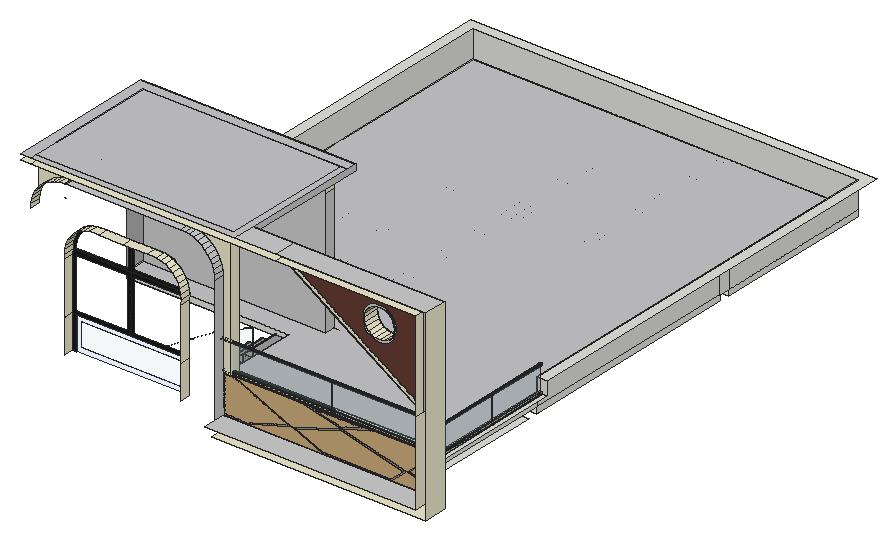
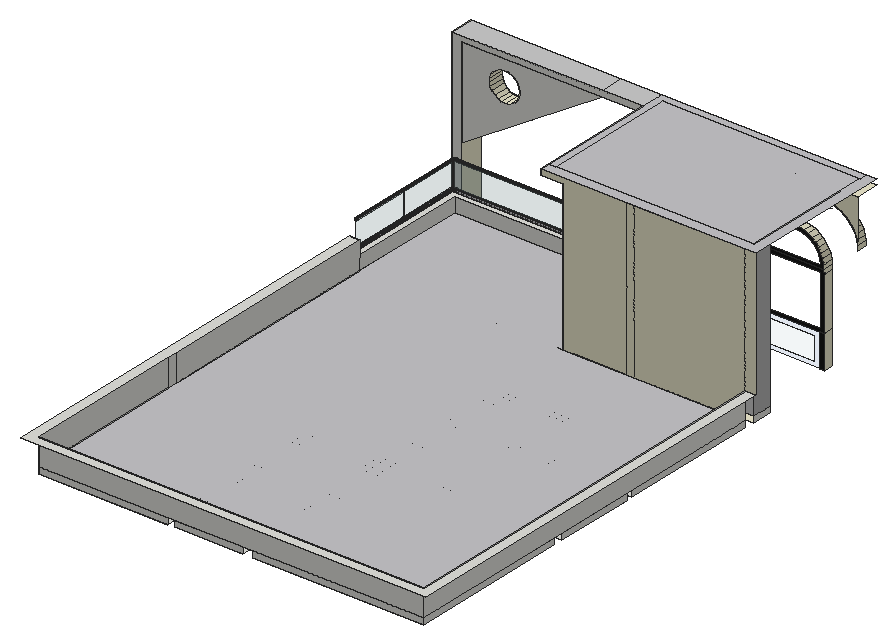
# SketchUp Ruby script. Lengths in inches.
U = 1.inch
M = Sketchup.active_model
def pt(a) = Geom::Point3d.new(a.map { |v| v * U })
def face(e, loops, mat)
  f = e.add_face(loops[0].map { |a| pt(a) })
  loops[1..].each { |l| e.add_face(l.map { |a| pt(a) }).erase! }
  f.material = f.back_material = mat if mat
  f
end
# faces: each face lists its corners as indices into pts; further lists are holes
def faces(e, pts, list, mat = nil) = list.each { |f| face(e, (f[0].is_a?(Array) ? f : [f]).map { |l| l.map { |i| pts[i] } }, mat) }
# xy, xz, yz: faces in a plane at the given z, y or x. An outline is a flat list of corners, or four numbers for a rectangle; further outlines are holes
def ring(l) = l.size == 4 ? [[l[0], l[1]], [l[2], l[1]], [l[2], l[3]], [l[0], l[3]]] : l.each_slice(2).to_a
def flat(e, list, mat, &to3) = list.each { |f| face(e, (f[0].is_a?(Array) ? f : [f]).map { |l| ring(l).map { |u, v| to3.(u, v) } }, mat) }
def xy(e, z, list, mat = nil) = flat(e, list, mat) { |x, y| [x, y, z] }
def xz(e, y, list, mat = nil) = flat(e, list, mat) { |x, z| [x, y, z] }
def yz(e, x, list, mat = nil) = flat(e, list, mat) { |y, z| [x, y, z] }
def lines(e, pts, list) = list.each { |a, b| e.add_line(pt(pts[a]), pt(pts[b])) }
# prism: a flat outline (further loops are holes) pulled along v
def prism(e, loops, v, mat = nil)
  f = face(e, loops, mat); d = Geom::Vector3d.new(v.map { |x| x * U })
  f.pushpull(f.normal.samedirection?(d) ? d.length : -d.length)
end
def box(e, o, s, mat = nil) = prism(e, [[o, [o[0] + s[0], o[1], o[2]], [o[0] + s[0], o[1] + s[1], o[2]], [o[0], o[1] + s[1], o[2]]]], [0, 0, s[2]], mat)
def at(x, y, z, deg = 0) = Geom::Transformation.translation(pt([x, y, z])) * Geom::Transformation.rotation(ORIGIN, Z_AXIS, deg.degrees)
def axes(o, x, y, z) = Geom::Transformation.new([*x, 0, *y, 0, *z, 0, *pt(o).to_a, 1])
def part(name) = M.definitions.add(name)
# library, detail: a bought-in or finely detailed component or shape, given as its bounding box
def library(name, o, s) = part(name).tap { |d| box(d.entities, o, s) }
def detail(e, o, s) = box(e.add_group.entities, o, s)
def put(e, d, t, mat = nil) = e.add_instance(d, t).tap { |i| i.material = mat if mat }
def group(e, t, mat = nil) = e.add_group.tap { |g| g.transformation = t; g.material = mat if mat }.entities
root = M.entities
M.materials.add("Copper (DK9VGZ)").color = [173, 110, 84]
M.materials.add("Distressed Leather (CCZUWY)").color = [102, 60, 53]
M.materials.add("Drag Textured Plaster None 1500 x 1662 mm (I93S2X)").color = [206, 173, 125]
M.materials.add("Drag Textured Plaster None 1500 x 1662 mm (TE616Y)").color = [206, 173, 125]
M.materials.add("Grey4").color = [61, 61, 61]
M.materials.add("Lily_Blonde").color = [237, 233, 206]
M.materials.add("Rosso Verona Marble Herringbone 1146 x 891 mm (N04GW4)").color = [204, 94, 55]
M.materials.add("Rust-Stain-Remover").color = [206, 203, 196]
M.materials["Rust-Stain-Remover"].alpha = 0.13
M.materials.add("Textured Stucco (8DUEUS)").color = [204, 204, 204]
M.materials.add("Wood Wool (CH8A6D)").color = [158, 148, 138]
M.materials.add("[0136_Charcoal]").color = [25, 25, 25]
M.materials.add("[Aluminum]").color = [178, 178, 178]
M.materials.add("[Metal Silver]").color = [198, 197, 201]
M.materials.add("[Metal Silver]1").color = [234, 233, 238]
M.materials.add("[Translucent Glass Blue]1").color = [97, 145, 232]
M.materials["[Translucent Glass Blue]1"].alpha = 0.15
M.materials.add("[Translucent Glass Gray]").color = [73, 161, 170]
M.materials["[Translucent Glass Gray]"].alpha = 0.06
M.materials.add("crushed-stone-asphalt-staggered-isosceles-2423-mm-architextu").color = [158, 158, 157]
c1 = part("Stair tread")
xy(c1.entities,0,[[0,0,11.5,36]])
xy(c1.entities,7,[[0,0,11.5,36]])
xz(c1.entities,0,[[0,0,11.5,7],[11.5,6,11.63,6.02,11.75,6.07,11.85,6.15,11.93,6.25,11.98,6.37,12,6.5,11.98,6.63,11.93,6.75,11.85,6.85,11.75,6.93,11.63,6.98,11.5,7]])
xz(c1.entities,36,[[0,0,11.5,7],[11.5,6,11.5,7,11.63,6.98,11.75,6.93,11.85,6.85,11.93,6.75,11.98,6.63,12,6.5,11.98,6.37,11.93,6.25,11.85,6.15,11.75,6.07,11.63,6.02]])
yz(c1.entities,0,[[0,0,36,7]])
yz(c1.entities,11.5,[[0,0,36,6],[0,6,10.3125,7],[10.3125,6,36,7]])
p = [[11.5,36,6],[11.63,36,6.02],[11.63,0,6.02],[11.5,0,6],[11.5,10.3125,6],[11.75,36,6.07],
  [11.75,0,6.07],[11.85,36,6.15],[11.85,0,6.15],[11.93,36,6.25],[11.93,0,6.25],[11.98,36,6.37],
  [11.98,0,6.37],[12,36,6.5],[12,0,6.5],[11.98,36,6.63],[11.98,0,6.63],[11.93,36,6.75],
  [11.93,0,6.75],[11.85,36,6.85],[11.85,0,6.85],[11.75,36,6.93],[11.63,36,6.98],[11.63,0,6.98],
  [11.75,0,6.93],[11.5,36,7],[11.5,10.3125,7],[11.5,0,7]]
faces(c1.entities,p,[[0,1,2,3,4],[1,5,6,2],[5,7,8,6],[7,9,10,8],[9,11,12,10],[11,13,14,12],[13,15,16,14],[15,17,18,16],
  [17,19,20,18],[21,22,23,24],[19,21,24,20],[25,26,27,23,22]])
c2 = part("Группа\#2")
box(c2.entities,[0,0,0],[41.85,0.39,23.61])
c3 = part("Группа\#3")
prism(c3.entities,[[[0,1.0625,0],[0,0.09,0],[0,0,0.09],[0,0,0.56],[0,0.2,0.66],[0,0.06,0.66],[0,0,0.72],[0,0,2.28],[0,0.4,2.69],[0,0.74,2.69],[0,0.74,1.08],[0,1.0625,1.08],[0,1.39,1.08],[0,1.39,2.69],[0,1.6875,2.69],[0,1.85,2.48],[0,1.85,0.09],[0,1.76,0]]],[41.85,0,0])
c4 = part("Группа\#4")
xy(c4.entities,0,[[0,0.06,41.85,0.58]],"[0136_Charcoal]")
xy(c4.entities,0.12,[[0,0.11,41.85,0.54]],"[Metal Silver]1")
xz(c4.entities,0,[[0,0.06,41.85,1.61]],"[0136_Charcoal]")
xz(c4.entities,0.11,[[0,0.12,41.85,1.67]],"[0136_Charcoal]")
xz(c4.entities,0.54,[[0,0.12,41.85,1.67]],"[0136_Charcoal]")
xz(c4.entities,0.65,[[0,0.07,41.85,1.61]],"[0136_Charcoal]")
yz(c4.entities,0,[[0.06,0,0,0.06,0,1.61,0.11,1.67,0.11,0.12,0.54,0.12,0.54,1.67,0.65,1.61,0.65,0.07,0.58,0]],"[0136_Charcoal]")
yz(c4.entities,41.85,[[0.06,0,0.58,0,0.65,0.07,0.65,1.61,0.54,1.67,0.54,0.12,0.11,0.12,0.11,1.67,0,1.61,0,0.06]],"[0136_Charcoal]")
p = [[41.85,0.06,0],[41.85,0,0.06],[0,0,0.06],[0,0.06,0],[41.85,0.65,0.07],[41.85,0.58,0],
  [0,0.58,0],[0,0.65,0.07],[41.85,0,1.61],[41.85,0.11,1.67],[0,0.11,1.67],[0,0,1.61],
  [41.85,0.54,1.67],[41.85,0.65,1.61],[0,0.65,1.61],[0,0.54,1.67]]
faces(c4.entities,p,[[0,1,2,3],[4,5,6,7],[8,9,10,11],[12,13,14,15]],"[0136_Charcoal]")
c5 = part("Группа\#5")
prism(c5.entities,[[[0,0.73,0],[0,0.49,0.1],[0,0.29,0.25],[0,0.13,0.46],[0,0.03,0.7],[0,0,0.95],[0,0.03,1.21],[0,0.13,1.44],[0,0.29,1.65],[0,0.49,1.8],[0,0.73,1.9],[0,0.98,1.93],[0,1.24,1.9],[0,1.48,1.8],[0,1.68,1.65],[0,1.84,1.44],[0,1.93,1.21],[0,1.97,0.95],[0,1.93,0.7],[0,1.84,0.46],[0,1.68,0.25],[0,1.48,0.1],[0,1.24,0],[0,1.24,0.55],[0,0.73,0.55]]],[83.93,0,0])
c6 = part("Группа\#1")
xz(c6.entities,0,[[0,0,41.85,23.61]],"Rust-Stain-Remover")
c7 = part("Группа\#6")
xz(c7.entities,0,[[0,0,41.85,23.61]],"Rust-Stain-Remover")
c8 = part("Перила_14")
put(c8.entities,c2,at(0,-0.2,1.22),"[Translucent Glass Gray]")
put(c8.entities,c3,at(0,-1.0625,0),"[Metal Silver]")
put(c8.entities,c4,at(0,-0.32,1.08))
put(c8.entities,c5,at(0,-0.98,24.31),"[Metal Silver]1")
put(c8.entities,c6,at(0,0,1.22))
put(c8.entities,c4,at(42.09,-0.32,1.08))
put(c8.entities,c2,at(42.09,-0.2,1.22),"[Translucent Glass Gray]")
put(c8.entities,c3,at(42.09,-1.0625,0),"[Metal Silver]")
put(c8.entities,c7,at(42.09,0,1.22))
xy(root,132.6875,[[163.71,20.75,281.1875,29.1875]])
xy(root,132.8125,[[169.71,0,360,20.75]],"Lily_Blonde")
xy(root,138.8125,[[163.71,0,351.58,20.75]],"Textured Stucco (8DUEUS)")
xy(root,156,[[163.71,29.1875,163.71,29.25,152.42,29.25,152.42,125.1875,351,125.1875,351,29.1875],[9,134.1875,9,260.1875,78,260.1875,78,266.1875,9,266.1875,9,338.1875,108,338.1875,108,260.1875,170,260.1875,170,302.1875,161,302.1875,161,266.1875,114,266.1875,114,338.1875,161,338.1875,161,332.1875,170,332.1875,170,338.1875,176,338.1875,176,347.1875,170,347.1875,170,353.1875,161,353.1875,161,347.1875,9,347.1875,9,491.1875,161,491.1875,161,395.1875,170,395.1875,170,416.1875,230,416.1875,230,395.1875,236,395.1875,236,455.1875,230,455.1875,230,422.1875,170,422.1875,170,491.1875,230,491.1875,230,485.1875,236,485.1875,236,491.1875,351,491.1875,351,347.1875,236,347.1875,236,353.1875,230,353.1875,230,338.1875,351,338.1875,351,134.1875,170,134.1875,170,224.1875,161,224.1875,161,213.1875,155,213.1875,155,207.1875,161,207.1875,161,134.1875,114,134.1875,114,207.1875,120,207.1875,120,213.1875,108,213.1875,108,134.1875]])
xy(root,156,[[9,107.1875,152.42,125.1875]],"Lily_Blonde")
xy(root,157.02,[[140.92,70.6875,149.67,71.1875]])
xy(root,161,[[163.71,29.1875,351,29.1875,351,491.1875,9,491.1875,9,134.1875,170.71,134.1875,170.71,125.1875,9,125.1875,9,107.1875,152.42,107.1875,152.42,29.25,163.71,29.25]],"[Metal Silver]")
xy(root,173,[[163.71,20.75,170.71,29.1875],[170.71,20.75,360,20.75,360,134.1875,351,134.1875,351,29.1875,170.71,29.1875]])
xy(root,173,[[163.71,20.1875,170.71,20.75]],"Grey4")
xy(root,185,[[0,134.1875,9,134.1875,9,491.1875,351,491.1875,351,134.1875,360,134.1875,360,500.1875,0,500.1875]])
xy(root,250,[[52.44,11.4375,60.625,20.1875],[60.625,11.4375,82.18,20.1875],[82.18,11.4375,103.73,20.1875],[103.73,11.4375,111.91,20.1875]],"Lily_Blonde")
xy(root,279.9375,[[154.71,29.1875,152,125.1875,170.71,125.1875,170.71,29.1875]])
xy(root,280,[[30,11.4375,30.32,20.1875],[30.32,11.4375,31.32,20.1875]],"Copper (DK9VGZ)")
xy(root,280,[[31.32,11.4375,133.71,20.1875]],"Textured Stucco (8DUEUS)")
xy(root,293,[[9,29.1875,9,125.1875,152,125.1875,154.71,29.1875]])
xy(root,293,[[0,0,9,20.1875],[9,0,226.71,20.1875],[226.71,0,351.58,6.9375],[170.71,20.1875,170.71,134.1875,190.71,134.1875,190.71,20.75,226.71,20.75,226.71,20.1875]],"Lily_Blonde")
xy(root,293,[[226.71,6.9375,351.58,20.75]],"Textured Stucco (8DUEUS)")
xy(root,298,[[190.71,0,226.71,20.75],[226.71,0,360,20.75]],"Textured Stucco (8DUEUS)")
xy(root,298,[[0,0,9,0,9,125.1875,190.71,125.1875,190.71,134.1875,0,134.1875],[9,0,190.71,0,190.71,125.1875,184.71,125.1875,184.71,6,9,6],[9,6,184.71,125.1875]],"[Metal Silver]")
xz(root,6.9375,[[[348.16,218.71,348.16,289.58,238.32,289.58],[312.95,255,309.01,255.67,305.37,257.33,302.29,259.88,299.98,263.14,298.59,266.89,298.22,270.87,298.89,274.8125,300.56,278.45,303.11,281.52,306.37,283.84,310.11,285.23,314.09,285.6,318.03,284.93,321.67,283.26,324.75,280.71,327.06,277.45,328.45,273.7,328.82,269.72,328.15,265.78,326.49,262.15,323.93,259.07,320.67,256.76,316.93,255.37]]],"Distressed Leather (CCZUWY)")
xz(root,6.9375,[[[351.58,212.4375,351.58,293,226.71,293,289.14,252.72],[348.16,218.71,238.32,289.58,348.16,289.58]]],"Lily_Blonde")
xz(root,6.9375,[[[312.95,255,316.93,255.37,320.67,256.76,323.93,259.07,326.49,262.15,328.15,265.78,328.82,269.72,328.45,273.7,327.06,277.45,324.75,280.71,321.67,283.26,318.03,284.93,314.09,285.6,310.11,285.23,306.37,283.84,303.11,281.52,300.56,278.45,298.89,274.8125,298.22,270.87,298.59,266.89,299.98,263.14,302.29,259.88,305.37,257.33,309.01,255.67],[313.02,256.93,309.58,257.51,306.4,258.97,303.71,261.2,301.69,264.05,300.48,267.32,300.15,270.8,300.74,274.24,302.19,277.42,304.42,280.11,307.27,282.13,310.54,283.34,314.02,283.67,317.46,283.08,320.64,281.625,323.33,279.4,325.35,276.55,326.5625,273.27,326.89,269.8,326.31,266.35,324.85,263.18,322.62,260.49,319.77,258.47,316.5,257.25]]],"Textured Stucco (8DUEUS)")
xz(root,20.1875,[[163.71,173,170.71,173,170.71,293,0,293,0,250,0.26,253.92,1.02,257.76,2.28,261.48,4.02,265,6.2,268.26,8.79,271.21,11.74,273.8,15,275.98,18.52,277.72,22.24,278.98,26.08,279.74,30,280,133.71,280,137.625,279.74,141.47,278.98,145.1875,277.72,148.71,275.98,151.97,273.8,154.92,271.21,157.51,268.26,159.6875,265,161.42,261.48,162.69,257.76,163.45,253.92,163.71,250]],"Lily_Blonde")
xz(root,20.1875,[[30,144,33.9,173],[130.23,144,133.71,173],[[30,173,82.18,173,82.18,224.1,30.32,224.1,30,220],[33.15,176.15,33.15,219.875,33.24,220.95,79.02,220.95,79.02,176.15]],[[82.18,173,133.71,173,133.71,220,134.03,224.1,82.18,224.1],[85.05,175.87,85.05,221.23,130.92,221.23,130.84,220.11,130.84,175.87]],[[30.32,224.1,82.18,224.1,82.18,250,52.44,250,48.44,249.04,44.64,247.47,41.13,245.32,38,242.65,35.33,239.52,33.18,236.01,31.61,232.21,30.65,228.2],[32.64,226.25,32.77,227.87,33.65,231.54,35.1,235.03,37.07,238.25,39.52,241.125,42.4,243.58,45.62,245.55,49.11,247,52.7,247.86,80.03,247.86,80.03,226.25]],
  [[82.18,224.1,134.03,224.1,133.71,228.2,132.75,232.21,131.18,236.01,129.03,239.52,126.35,242.65,123.22,245.32,119.72,247.47,115.91,249.04,111.91,250,82.18,250],[84.45,226.375,84.45,247.73,111.64,247.73,115.21,246.875,118.68,245.4375,121.88,243.47,124.74,241.03,127.18,238.18,129.14,234.97,130.58,231.5,131.46,227.85,131.57,226.375]]],"[0136_Charcoal]")
xz(root,20.1875,[[[33.9,144,130.23,173],[38.1875,148.28,125.95,168.72]]],"[Translucent Glass Blue]1")
xz(root,20.1875,[[38.1875,148.28,125.95,168.72]],"[Translucent Glass Gray]")
xz(root,20.75,[[351.58,173,351.58,293,190.71,293,190.71,298,360,298,360,173],[[351.58,212.4375,289.14,252.72,226.71,293,351.58,293],[313.02,256.93,316.5,257.25,319.77,258.47,322.62,260.49,324.85,263.18,326.31,266.35,326.89,269.8,326.5625,273.27,325.35,276.55,323.33,279.4,320.64,281.625,317.46,283.08,314.02,283.67,310.54,283.34,307.27,282.13,304.42,280.11,302.19,277.42,300.74,274.24,300.15,270.8,300.48,267.32,301.69,264.05,303.71,261.2,306.4,258.97,309.58,257.51]]])
xz(root,20.75,[[184.63,138.8125,251.86,138.8125,224.17,150.92],[313.3,138.8125,351.58,138.8125,351.58,144.47,326.39,150.51],[164.7,139.81,184.48,139.81,221.3,151.09,173.46,172,164.7,172],[252.17,140.28,312.74,140.28,323.33,149.74,268.34,162.92,228.38,150.68],[350.65,145.65,350.65,170.93,328.33,151],
  [326.39,150.51,351.58,173,296.25,173,268.29,164.4375],[224.17,150.92,268.29,164.4375,232.57,173,173.67,173],[268.25,165.77,287.63,171.71,243.49,171.71]],"Drag Textured Plaster None 1500 x 1662 mm (I93S2X)")
xz(root,20.75,[[163.71,132.6875,169.71,132.6875,169.71,132.8125,360,132.8125,360,173,351.58,173,351.58,138.8125,163.71,138.8125]],"Drag Textured Plaster None 1500 x 1662 mm (TE616Y)")
xz(root,20.75,[[[163.71,138.8125,184.63,138.8125,224.17,150.92,173.67,173,163.71,173],[164.7,139.81,164.7,172,173.46,172,221.3,151.09,184.48,139.81]],[[251.86,138.8125,313.3,138.8125,326.39,150.51,268.29,164.4375,224.17,150.92],[252.17,140.28,228.38,150.68,268.34,162.92,323.33,149.74,312.74,140.28]],[[351.58,144.47,351.58,173,326.39,150.51],[350.65,145.65,328.33,151,350.65,170.93]],[[268.29,164.4375,296.25,173,232.57,173],[268.25,165.77,243.49,171.71,287.63,171.71]]],"Wood Wool (CH8A6D)")
xz(root,29.1875,[[163.71,132.6875,351,156],[163.71,161,351,173]])
xz(root,29.1875,[[163.71,173,170.71,279.9375]],"Grey4")
xz(root,29.25,[[152.42,156,163.71,161]])
xz(root,70.6875,[[117.92,143.04,140.92,157.02,149.67,157.02,149.67,181.02,117.92,167.02]],"[Translucent Glass Gray]")
xz(root,107.1875,[[9,156,152.42,161]])
xz(root,125.1875,[[9,161,170.71,161,170.71,279.9375,152,279.9375,152,293,9,293]],"Textured Stucco (8DUEUS)")
xz(root,134.1875,[[9,156,108,161],[114,156,161,161],[351,173,360,185]])
xz(root,134.1875,[[9,161,108,298],[108,161,114,298],[114,161,114,298,190.71,298,190.71,293,170.71,293,170.71,161],[0,185,9,298]],"Lily_Blonde")
xz(root,491.1875,[[9,156,161,161],[170,156,230,161],[236,156,351,161],[9,161,351,185]])
yz(root,9,[[107.1875,156,125.1875,161],[134.1875,156,260.1875,161],[266.1875,156,338.1875,161],[347.1875,156,491.1875,161],[134.1875,161,491.1875,185],
  [29.1875,293,107.1875,298],[107.1875,293,125.1875,298]])
yz(root,9,[[107.1875,161,125.1875,293]],"[Aluminum]")
yz(root,30,[[11.4375,144,20.1875,173],[11.4375,173,20.1875,220]],"Lily_Blonde")
yz(root,133.71,[[11.4375,144,20.1875,173],[11.4375,173,20.1875,220]],"Lily_Blonde")
yz(root,149.67,[[70.6875,157.02,71.1875,181.02]])
yz(root,152.42,[[29.25,156,107.1875,157.02],[29.25,157.02,107.1875,161]])
yz(root,163.71,[[20.75,144.15,29.1875,173],[29.1875,156,29.25,161]])
yz(root,163.71,[[20.75,132.6875,29.1875,144.15]],"Rosso Verona Marble Herringbone 1146 x 891 mm (N04GW4)")
yz(root,163.71,[[11.4375,138.8125,20.75,138.8125,20.75,173,20.1875,173,20.1875,250,11.4375,250]],"Textured Stucco (8DUEUS)")
yz(root,170.71,[[20.1875,173,29.1875,173,29.1875,279.9375,125.1875,279.9375,125.1875,271.4375,134.1875,271.4375,134.1875,293,20.1875,293]],"Lily_Blonde")
yz(root,170.71,[[125.1875,161,134.1875,271.4375]],"Textured Stucco (8DUEUS)")
yz(root,190.71,[[20.75,293,134.1875,298]],"Textured Stucco (8DUEUS)")
yz(root,351,[[134.1875,156,338.1875,161],[347.1875,156,491.1875,161],[29.1875,161,134.1875,173],[134.1875,161,338.1875,185],[338.1875,161,347.1875,185],
  [347.1875,161,491.1875,185]])
yz(root,351.58,[[0,138.8125,20.75,212.4375],[0,212.4375,6.9375,293]],"Lily_Blonde")
yz(root,351.58,[[6.9375,212.4375,20.75,293]],"Textured Stucco (8DUEUS)")
yz(root,360,[[0,132.8125,20.75,298]],"Lily_Blonde")
p = [[94.82,71.1875,153],[71.92,71.1875,139.02],[71.92,70.6875,139.02],[94.82,70.6875,153],[117.92,71.1875,143.04],[140.92,71.1875,157.02],
  [140.92,70.6875,157.02],[117.92,70.6875,143.04],[117.92,71.1875,167.02],[117.92,70.6875,167.02],[149.67,71.1875,181.02],[149.67,70.6875,181.02],
  [351.58,6.9375,212.4375],[289.14,6.9375,252.72],[289.14,20.75,252.72],[351.58,20.75,212.4375],[30,20.1875,220],[30.32,20.1875,224.1],
  [30.32,11.4375,224.1],[30,11.4375,220],[134.03,20.1875,224.1],[133.71,20.1875,220],[133.71,11.4375,220],[134.03,11.4375,224.1],
  [30.65,20.1875,228.2],[30.65,11.4375,228.2],[133.71,20.1875,228.2],[133.71,11.4375,228.2],[31.61,20.1875,232.21],[31.61,11.4375,232.21],
  [132.75,20.1875,232.21],[132.75,11.4375,232.21],[33.18,20.1875,236.01],[33.18,11.4375,236.01],[131.18,20.1875,236.01],[131.18,11.4375,236.01],
  [35.33,20.1875,239.52],[35.33,11.4375,239.52],[129.03,20.1875,239.52],[129.03,11.4375,239.52],[38,20.1875,242.65],[38,11.4375,242.65],
  [126.35,20.1875,242.65],[126.35,11.4375,242.65],[41.13,20.1875,245.32],[41.13,11.4375,245.32],[123.22,20.1875,245.32],[123.22,11.4375,245.32],
  [44.64,20.1875,247.47],[44.64,11.4375,247.47],[119.72,20.1875,247.47],[119.72,11.4375,247.47],[48.44,20.1875,249.04],[48.44,11.4375,249.04],
  [115.91,20.1875,249.04],[115.91,11.4375,249.04],[52.44,20.1875,250],[52.44,11.4375,250],[111.91,20.1875,250],[111.91,11.4375,250],
  [0.26,20.1875,253.92],[0,20.1875,250],[0,11.4375,250],[0.26,11.4375,253.92],[163.71,20.1875,250],[163.45,20.1875,253.92],
  [163.45,11.4375,253.92],[163.71,11.4375,250],[226.71,20.75,293],[226.71,6.9375,293],[226.71,20.1875,293],[1.02,20.1875,257.76],
  [1.02,11.4375,257.76],[162.69,20.1875,257.76],[162.69,11.4375,257.76],[309.58,6.9375,257.51],[313.02,6.9375,256.93],[313.02,20.75,256.93],
  [309.58,20.75,257.51],[316.5,6.9375,257.25],[316.5,20.75,257.25],[319.77,6.9375,258.47],[319.77,20.75,258.47],[306.4,6.9375,258.97],
  [306.4,20.75,258.97],[2.28,20.1875,261.48],[2.28,11.4375,261.48],[161.42,20.1875,261.48],[161.42,11.4375,261.48],[322.62,6.9375,260.49],
  [322.62,20.75,260.49],[303.71,6.9375,261.2],[303.71,20.75,261.2],[324.85,6.9375,263.18],[324.85,20.75,263.18],[301.69,6.9375,264.05],
  [301.69,20.75,264.05],[4.02,20.1875,265],[4.02,11.4375,265],[159.6875,20.1875,265],[159.6875,11.4375,265],[326.31,6.9375,266.35],
  [326.31,20.75,266.35],[300.48,6.9375,267.32],[300.48,20.75,267.32],[6.2,20.1875,268.26],[6.2,11.4375,268.26],[157.51,20.1875,268.26],
  [157.51,11.4375,268.26],[326.89,6.9375,269.8],[326.89,20.75,269.8],[300.15,6.9375,270.8],[300.15,20.75,270.8],[8.79,20.1875,271.21],
  [8.79,11.4375,271.21],[154.92,20.1875,271.21],[154.92,11.4375,271.21],[326.5625,6.9375,273.27],[326.5625,20.75,273.27],[300.74,6.9375,274.24],
  [300.74,20.75,274.24],[11.74,20.1875,273.8],[11.74,11.4375,273.8],[151.97,20.1875,273.8],[151.97,11.4375,273.8],[325.35,6.9375,276.55],
  [325.35,20.75,276.55],[15,20.1875,275.98],[15,11.4375,275.98],[148.71,20.1875,275.98],[148.71,11.4375,275.98],[302.19,6.9375,277.42],
  [302.19,20.75,277.42],[18.52,20.1875,277.72],[18.52,11.4375,277.72],[145.1875,20.1875,277.72],[145.1875,11.4375,277.72],[323.33,6.9375,279.4],
  [323.33,20.75,279.4],[304.42,6.9375,280.11],[304.42,20.75,280.11],[22.24,20.1875,278.98],[22.24,11.4375,278.98],[141.47,20.1875,278.98],
  [141.47,11.4375,278.98],[26.08,20.1875,279.74],[26.08,11.4375,279.74],[137.625,20.1875,279.74],[137.625,11.4375,279.74],[320.64,6.9375,281.625],
  [320.64,20.75,281.625],[30,20.1875,280],[30,11.4375,280],[133.71,20.1875,280],[133.71,11.4375,280],[154.71,29.1875,293],
  [152,125.1875,293],[152,125.1875,279.9375],[154.71,29.1875,279.9375],[307.27,6.9375,282.13],[307.27,20.75,282.13],[317.46,6.9375,283.08],
  [317.46,20.75,283.08],[310.54,6.9375,283.34],[310.54,20.75,283.34],[314.02,6.9375,283.67],[314.02,20.75,283.67],[161,207.1875,156],
  [161,207.1875,161],[114,207.1875,156],[114,207.1875,161],[120,207.1875,156],[120,207.1875,161],[120,213.1875,156],
  [120,213.1875,161],[114,213.1875,156],[114,213.1875,161],[108,213.1875,156],[108,213.1875,161],[108,207.1875,156],
  [108,207.1875,161],[78,260.1875,156],[78,260.1875,161],[78,266.1875,156],[78,266.1875,161],[108,338.1875,156],
  [108,338.1875,161],[108,260.1875,156],[108,260.1875,161],[170,260.1875,156],[170,260.1875,161],[170,302.1875,156],
  [170,302.1875,161],[161,302.1875,156],[161,302.1875,161],[161,266.1875,156],[161,266.1875,161],[114,266.1875,156],
  [114,266.1875,161],[114,338.1875,156],[114,338.1875,161],[161,338.1875,156],[161,338.1875,161],[161,332.1875,156],
  [161,332.1875,161],[170,332.1875,156],[170,332.1875,161],[170,338.1875,156],[170,338.1875,161],[176,338.1875,156],
  [176,338.1875,161],[176,347.1875,156],[176,347.1875,161],[170,347.1875,156],[170,347.1875,161],[170,353.1875,156],
  [170,353.1875,161],[161,353.1875,156],[161,353.1875,161],[161,347.1875,156],[161,347.1875,161],[161,395.1875,156],
  [161,395.1875,161],[170,395.1875,156],[170,395.1875,161],[170,416.1875,156],[170,416.1875,161],[230,416.1875,156],
  [230,416.1875,161],[230,395.1875,156],[230,395.1875,161],[236,395.1875,156],[236,395.1875,161],[236,455.1875,156],
  [236,455.1875,161],[230,455.1875,156],[230,455.1875,161],[230,422.1875,156],[230,422.1875,161],[170,422.1875,156],
  [170,422.1875,161],[230,485.1875,156],[230,485.1875,161],[236,485.1875,156],[236,485.1875,161],[236,347.1875,156],
  [236,347.1875,161],[236,353.1875,156],[236,353.1875,161],[230,353.1875,156],[230,353.1875,161],[230,338.1875,156],
  [230,338.1875,161],[230,134.1875,156],[230,134.1875,161],[176,134.1875,156],[176,134.1875,161],[170,134.1875,156],
  [170,134.1875,161],[170,224.1875,156],[170,224.1875,161],[161,224.1875,156],[161,224.1875,161],[161,213.1875,156],
  [161,213.1875,161],[155,213.1875,156],[155,213.1875,161],[155,207.1875,156],[155,207.1875,161],[48.42,29.1875,293],
  [48.42,29.1875,298],[103.73,20.1875,250],[103.71,20.1875,250],[60.625,20.1875,250],[60.65,20.1875,250],[9,29.1875,293],
  [9,20.1875,293],[163.9,20.1875,173.13],[163.71,21.54,173],[170.71,134.1875,161],[117.92,71.1875,143.02],[31.32,11.4375,268.98],
  [30,11.4375,268.98]]
faces(root,p,[[0,1,2,3],[4,5,6,7],[8,0,3,9],[10,8,9,11],[155,156,157,158]])
faces(root,p,[[12,13,14,15],[16,17,18,19],[20,21,22,23],[17,24,25,18],[26,20,23,27],[24,28,29,25],[30,26,27,31],[28,32,33,29],
  [34,30,31,35],[32,36,37,33],[38,34,35,39],[36,40,41,37],[42,38,39,43],[40,44,45,41],[46,42,43,47],[44,48,49,45],
  [50,46,47,51],[48,52,53,49],[54,50,51,55],[52,56,57,53],[58,54,55,59],[60,61,62,63],[68,14,13,69,70],[71,60,63,72],
  [75,76,77,78],[76,79,80,77],[79,81,82,80],[83,75,78,84],[85,71,72,86],[81,89,90,82],[91,83,84,92],[89,93,94,90],
  [95,91,92,96],[97,85,86,98],[93,101,102,94],[103,95,96,104],[105,97,98,106],[101,109,110,102],[111,103,104,112],[113,105,106,114],
  [109,117,118,110],[119,111,112,120],[121,113,114,122],[117,125,126,118],[127,121,122,128],[131,119,120,132],[133,127,128,134],[125,137,138,126],
  [139,131,132,140],[141,133,134,142],[145,141,142,146],[137,149,150,138],[151,145,146,152],[159,139,140,160],[149,161,162,150],[163,159,160,164],
  [161,165,166,162],[165,163,164,166]],"Lily_Blonde")
faces(root,p,[[64,65,66,67],[65,73,74,66],[73,87,88,74],[87,99,100,88],[99,107,108,100],[107,115,116,108],[115,123,124,116],[123,129,130,124],
  [129,135,136,130],[135,143,144,136],[143,147,148,144],[147,153,154,148]],"Textured Stucco (8DUEUS)")
lines(root,p,[[167,168],[169,170],[171,172],[173,174],[175,176],[177,178],[179,180],[181,182],[183,184],[185,186],[187,188],[189,190],
  [191,192],[193,194],[195,196],[197,198],[199,200],[201,202],[203,204],[205,206],[207,208],[209,210],[211,212],[213,214],
  [215,216],[217,218],[219,220],[221,222],[223,224],[225,226],[227,228],[229,230],[231,232],[233,234],[235,236],[237,238],
  [239,240],[241,242],[243,244],[245,246],[247,248],[249,250],[251,252],[253,254],[255,256],[257,258],[259,260],[261,262],
  [263,264],[265,266],[267,268],[269,270],[271,272],[273,274],[275,276],[64,277],[277,278],[256,279],[280,4],[281,282]])
put(root,c1,at(129.42,107.1875,136.02,-180),"crushed-stone-asphalt-staggered-isosceles-2423-mm-architextu")
put(root,c1,at(140.92,107.1875,143.02,-180),"crushed-stone-asphalt-staggered-isosceles-2423-mm-architextu")
put(root,c1,at(152.42,107.1875,150.02,-180),"crushed-stone-asphalt-staggered-isosceles-2423-mm-architextu")
put(root,c8,axes([160.81,22.6,173],[2.3346,0,0],[0,1,0],[0,0,1]),"Textured Stucco (8DUEUS)")
put(root,c8,axes([356.96,131.65,173.96],[0,-1.28716,0],[1,0,0],[0,0,0.97]))
